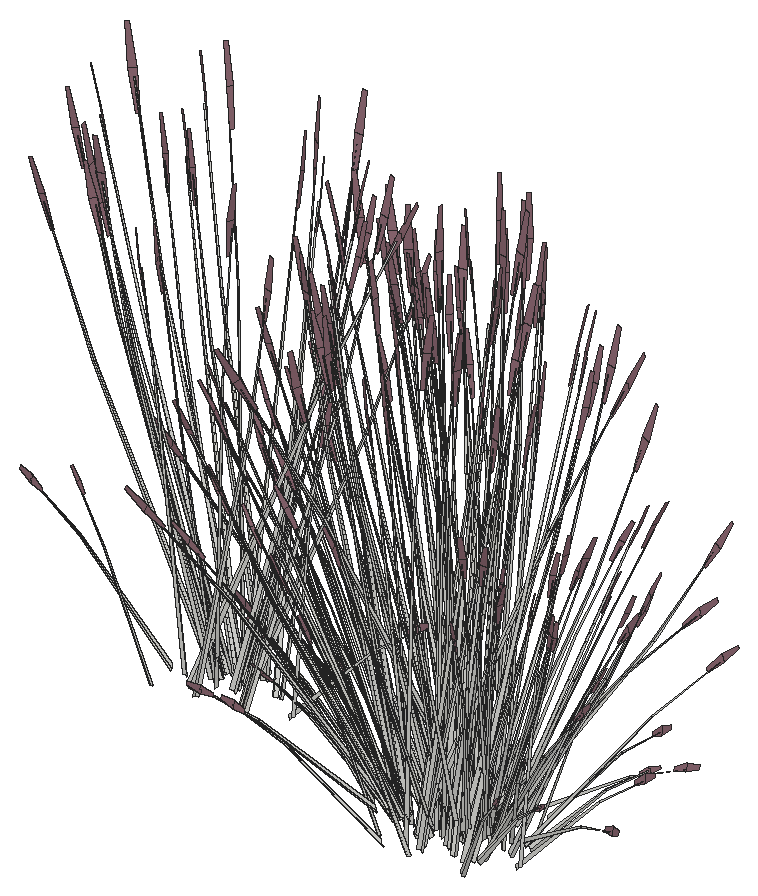
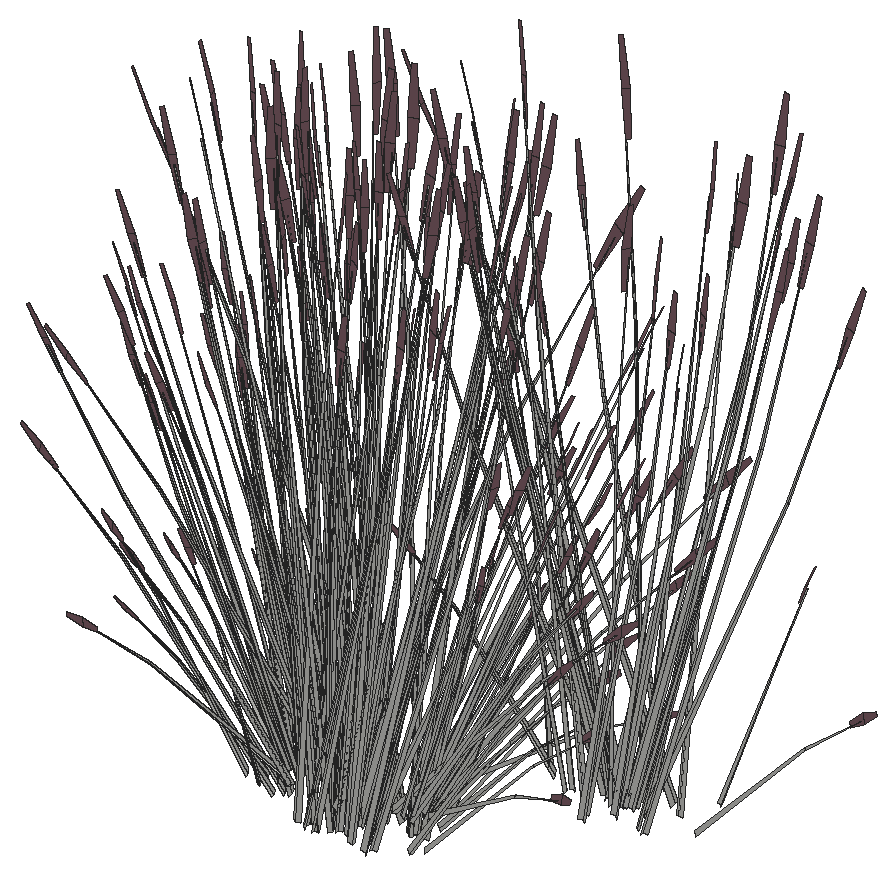
# SketchUp Ruby script. Lengths in inches.
U = 1.inch
M = Sketchup.active_model
def pt(a) = Geom::Point3d.new(a.map { |v| v * U })
def face(e, loops, mat)
  f = e.add_face(loops[0].map { |a| pt(a) })
  loops[1..].each { |l| e.add_face(l.map { |a| pt(a) }).erase! }
  f.material = f.back_material = mat if mat
  f
end
# faces: each face lists its corners as indices into pts; further lists are holes
def faces(e, pts, list, mat = nil) = list.each { |f| face(e, (f[0].is_a?(Array) ? f : [f]).map { |l| l.map { |i| pts[i] } }, mat) }
# xy, xz, yz: faces in a plane at the given z, y or x. An outline is a flat list of corners, or four numbers for a rectangle; further outlines are holes
def ring(l) = l.size == 4 ? [[l[0], l[1]], [l[2], l[1]], [l[2], l[3]], [l[0], l[3]]] : l.each_slice(2).to_a
def flat(e, list, mat, &to3) = list.each { |f| face(e, (f[0].is_a?(Array) ? f : [f]).map { |l| ring(l).map { |u, v| to3.(u, v) } }, mat) }
def xy(e, z, list, mat = nil) = flat(e, list, mat) { |x, y| [x, y, z] }
def xz(e, y, list, mat = nil) = flat(e, list, mat) { |x, z| [x, y, z] }
def yz(e, x, list, mat = nil) = flat(e, list, mat) { |y, z| [x, y, z] }
def lines(e, pts, list) = list.each { |a, b| e.add_line(pt(pts[a]), pt(pts[b])) }
# prism: a flat outline (further loops are holes) pulled along v
def prism(e, loops, v, mat = nil)
  f = face(e, loops, mat); d = Geom::Vector3d.new(v.map { |x| x * U })
  f.pushpull(f.normal.samedirection?(d) ? d.length : -d.length)
end
def box(e, o, s, mat = nil) = prism(e, [[o, [o[0] + s[0], o[1], o[2]], [o[0] + s[0], o[1] + s[1], o[2]], [o[0], o[1] + s[1], o[2]]]], [0, 0, s[2]], mat)
def at(x, y, z, deg = 0) = Geom::Transformation.translation(pt([x, y, z])) * Geom::Transformation.rotation(ORIGIN, Z_AXIS, deg.degrees)
def axes(o, x, y, z) = Geom::Transformation.new([*x, 0, *y, 0, *z, 0, *pt(o).to_a, 1])
def part(name) = M.definitions.add(name)
# library, detail: a bought-in or finely detailed component or shape, given as its bounding box
def library(name, o, s) = part(name).tap { |d| box(d.entities, o, s) }
def detail(e, o, s) = box(e.add_group.entities, o, s)
def put(e, d, t, mat = nil) = e.add_instance(d, t).tap { |i| i.material = mat if mat }
def group(e, t, mat = nil) = e.add_group.tap { |g| g.transformation = t; g.material = mat if mat }.entities
root = M.entities
M.materials.add("LightPink_Translucent").color = [144, 107, 117]
c1 = part("blade")
p = [[2.15,0.21,22],[0,0.17,0],[0.09,0.45,0],[2.18,0.31,22],[2.29,0.31,22],[0.38,0.45,0],
  [2.48,0.24,33],[2.49,0.24,33],[2.48,0.22,33]]
faces(c1.entities,p,[[0,1,2,3],[4,5,2,3],[6,3,4,7],[8,0,3,6]])
c2 = part("seeds")
p = [[0.3,-0.1,1.38],[-0.01,-0.03,1.59],[-0.01,-0.03,0.03],[0.14,-0.07,-0.07],[0.29,-0.03,3],[0.15,0.01,3.11]]
faces(c2.entities,p,[[0,1,2,3],[1,0,4,5]],"LightPink_Translucent")
c3 = part("blade with seeds")
put(c3.entities,c1,at(0,0,0))
put(c3.entities,c2,axes([2.4,0.25,30.99],[1.5799,-0.05474,1.17369],[-0.12525,1.92788,0.29478],[-0.07173,-0.02425,1.56792]))
put(root,c3,axes([73.51,642.17,38.52],[0.55698,-0.6579,0.0643],[0.79316,0.38303,0.50621],[-0.25643,-0.21093,0.77189]))
put(root,c3,axes([71.35,642.08,35.29],[-0.11871,0.13643,1.76342],[-1.19964,0.29415,-0.26939],[-0.2898,-0.26759,0.30037]))
put(root,c3,axes([73.33,645.83,35.89],[-0.50328,-1.06202,-0.69835],[1.44974,-0.38248,-0.18329],[-0.05563,-0.35963,1.54149]))
put(root,c3,axes([70.71,643.46,37.67],[0.45521,0.17844,1.71376],[-0.94204,0.74856,0.13857],[-0.58713,-0.33769,0.73262]))
put(root,c3,axes([80.0625,642.58,35.29],[-0.18342,-0.08159,1.76342],[-0.47115,-0.9115,-0.26939],[0.31784,-0.24736,0.30037]))
put(root,c3,axes([51.08,643.17,44.21],[0.59459,-0.93321,-0.44739],[1.23546,0.44912,0.21531],[0,-0.21512,1.43643]))
put(root,c3,axes([76.27,642.79,38.84],[-0.36946,0.79643,0.35414],[-1.07787,-0.23229,-0.4572],[-0.09883,-0.32066,0.87481]))
put(root,c3,axes([51.625,642.71,44.67],[-0.1428,-1.18174,-0.29095],[1.48733,-0.07145,-0.50002],[0.26191,-0.15741,1.59708]))
put(root,c3,axes([47.9375,642.77,44.03],[0.85545,-0.64616,-0.30978],[0.85545,0.64616,0.30978],[0,-0.20813,1.38974]))
put(root,c3,axes([72.91,642.93,38.47],[-1.20928,0.24619,-0.51099],[-0.21154,-0.93233,-0.3958],[-0.32481,-0.26718,0.97773]))
put(root,c3,axes([79.02,643.125,38.53],[0.87265,0.70663,0.48003],[-0.92674,0.60943,0.3958],[0.16097,-0.33153,0.9933]))
put(root,c3,axes([73.76,642.1,39.22],[-0.81789,0.99285,-0.13619],[-1.18445,-0.572,-0.75594],[-0.41173,-0.28051,1.14864]))
put(root,c3,axes([47.59,639.67,44.13],[-0.35352,0.84566,-0.03893],[-1.08806,-0.26014,-0.17649],[-0.1652,-0.13832,0.58215]))
put(root,c3,axes([79.35,643.19,38.52],[1.00708,0.04826,0.0643],[-0.02761,0.72867,0.50621],[0.10538,-0.27912,0.77189]))
put(root,c3,axes([50.93,643.95,44.67],[-1.38012,-0.49416,-0.29095],[0.66454,-1.04299,-0.50002],[-0.04337,-0.25608,1.59708]))
put(root,c3,axes([78.59,643.6875,38.84],[-0.82919,0.54528,0.35414],[-0.78493,-0.62262,-0.4572],[0.11943,-0.31634,0.87481]))
put(root,c3,axes([80.06,645.16,38.77],[0.64013,-0.81717,-0.71045],[1.12174,0.58074,0.08574],[0.38221,-0.29607,1.00501]))
put(root,c3,axes([51.43,640.09,44.03],[1.14332,0.25625,-0.30978],[-0.28787,0.90242,0.30978],[0.23049,-0.10406,1.38974]))
put(root,c3,axes([73.14,642.78,36.17],[-0.7662,-1.03778,0],[1.28187,-0.57875,-0.51607],[0.29196,-0.13181,1.63711]))
put(root,c3,axes([80.02,644.77,38.47],[-0.31482,-0.94565,-0.51099],[1.19224,-0.16542,-0.3958],[0.34166,-0.254,0.97773]))
put(root,c3,axes([74.82,641.53,35.92],[-0.84686,0.59414,-0.03893],[-0.77596,-0.65071,-0.17649],[-0.05463,-0.18438,0.58215]))
put(root,c3,axes([70.625,641.8125,38.51],[-0.26368,-0.00731,1.74944],[-0.83946,0.73103,-0.27667],[-0.44791,-0.14937,0.14031]))
put(root,c3,axes([80.59,645.45,38.83],[-1.1336,-0.57106,-0.1216],[0.65308,-0.827,-0.67495],[0.32027,-0.28747,1.02557]))
put(root,c3,axes([75.9,648.57,37.12],[1.05902,0.41762,1.51261],[-1.03748,0.89969,0.59816],[-0.46471,-0.53324,1.26806]))
put(root,c3,axes([73.68,642.92,38.84],[0.18927,0.83419,0.35414],[-1.08199,0.22027,-0.4572],[-0.29062,-0.23905,0.87481]))
put(root,c3,axes([70.37,645.68,35.8125],[0,-1.03566,-0.49651],[1.37109,0,0],[0,-0.23588,1.57504]))
put(root,c3,axes([74.18,642.62,35.8125],[1.14694,-0.51783,-0.49651],[0.68554,0.92854,0],[0.26122,-0.11794,1.57504]))
put(root,c3,axes([80.98,644.4,36.38],[-0.4378,-0.03068,1.43002],[-0.44851,-0.8229,-0.30754],[0.53783,-0.23279,0.61141]))
put(root,c3,axes([70.43,643.47,38.89],[1.01205,-0.7643,0.53763],[0.87284,0.81167,0.4433],[-0.47482,-0.14098,1.11249]))
put(root,c3,axes([83.38,645.2,38.5],[-0.16006,-0.00787,1.77383],[-0.66468,-0.8428,-0.16761],[0.26693,-0.27711,0.31391]))
put(root,c3,axes([75.54,644.74,35.85],[0.82544,-0.77843,-0.62353],[1.0254,0.70586,-0.16365],[0.33076,-0.19418,1.37633]))
put(root,c3,axes([51.28,645.04,44.4375],[0.32481,-1.2272,-0.23429],[1.54007,0.21392,0.51271],[-0.26911,-0.16947,1.5644]))
put(root,c3,axes([81.49,642.89,36.56],[-0.40819,0.5272,1.1486],[-0.35086,-0.70831,0.84392],[0.33713,-0.17749,0.25299]))
put(root,c3,axes([80.9,644.87,38.32],[1.06674,-0.14801,-0.35414],[0.28168,0.84611,0.4572],[0.30569,-0.22726,0.87481]))
put(root,c3,axes([70.89,643.46,38.52],[0.06171,-0.78753,0.0643],[0.9318,0.02159,0.50621],[-0.35694,-0.08241,0.77189]))
put(root,c3,axes([74.1,646.1,36],[0.59459,-0.93321,-0.44739],[1.23546,0.44912,0.21531],[0,-0.21512,1.43643]))
put(root,c3,axes([70.54,643.71,38.32],[-0.69728,-0.64842,-0.35414],[0.79619,-0.61382,0.4572],[-0.40453,-0.09339,0.87481]))
put(root,c3,axes([74.64,645.64,36.46],[-0.1428,-1.18174,-0.29095],[1.48733,-0.07145,-0.50002],[0.26191,-0.15741,1.59708]))
put(root,c3,axes([70.95,645.7,35.82],[0.85545,-0.64616,-0.30978],[0.85545,0.64616,0.30978],[0,-0.20813,1.38974]))
put(root,c3,axes([51.17,644.55,44.21],[-0.73619,-0.86927,-0.44739],[1.11511,-0.61213,0.21531],[-0.23824,-0.10756,1.43643]))
put(root,c3,axes([70.61,642.61,35.92],[-0.35352,0.84566,-0.03893],[-1.08806,-0.26014,-0.17649],[-0.1652,-0.13832,0.58215]))
put(root,c3,axes([80.03,645.37,38.84],[-1.06674,0.14801,0.35414],[-0.28168,-0.84611,-0.4572],[0.30569,-0.22726,0.87481]))
put(root,c3,axes([73.95,646.88,36.46],[-1.38012,-0.49416,-0.29095],[0.66454,-1.04299,-0.50002],[-0.04337,-0.25608,1.59708]))
put(root,c3,axes([70.02,646.47,36.17],[-1.53239,0,0],[0,-1.1575,-0.51607],[0,-0.26363,1.63711]))
put(root,c3,axes([60.21,643.33,44.26],[-0.75977,-0.66224,-0.06488],[0.83212,-0.6068,-0.29416],[0.23578,-0.04272,0.97024]))
put(root,c3,axes([70.29,644.4,36.38],[0.23927,0.28834,1.43002],[-0.55135,0.78376,-0.30754],[-0.56612,-0.18733,0.61141]))
put(root,c3,axes([74.45,643.02,35.82],[1.14332,0.25625,-0.30978],[-0.28787,0.90242,0.30978],[0.23049,-0.10406,1.38974]))
put(root,c3,axes([71.27,644.14,38.77],[-1.22504,-0.02494,-0.71045],[0.08228,-1.05005,0.08574],[-0.51899,-0.11081,1.00501]))
put(root,c3,axes([50.51,644.88,44.06],[-1.27479,-0.1698,-0.62353],[0.26901,-1.04736,-0.16365],[-0.38043,-0.12691,1.37633]))
put(root,c3,axes([81,645.24,38.52],[0.8413,0.43556,0.0643],[-0.48981,0.62025,0.50621],[0.26973,-0.20053,0.77189]))
put(root,c3,axes([80.77,645.06,38.53],[0.30393,0.95317,0.48003],[-1.19224,0.16542,0.3958],[0.35138,-0.22417,0.9933]))
put(root,c3,axes([83.98,646.21,38.51],[0.17006,-0.15775,1.74944],[-0.21766,-0.96766,-0.27667],[0.42669,-0.18347,0.14031]))
put(root,c3,axes([50.22,641.94,43.59],[-1.20625,0.41464,1.28929],[-0.38394,-1.1897,0.50096],[0.74071,0.01979,1.46642]))
put(root,c3,axes([71.21,646.16,36.125],[-1.1399,0.87071,0.30756],[-1.1406,-0.86155,-0.36492],[-0.03981,-0.24727,1.64885]))
put(root,c3,axes([69.61,642.43,38.5],[0.09085,0.10335,1.77383],[-0.43798,0.92907,-0.16761],[-0.44357,0.00672,0.31391]))
put(root,c3,axes([59.64,643.56,43.49],[-0.06405,-0.15723,1.76342],[0.44421,-0.91974,-0.26939],[0.4481,-0.01323,0.30037]))
put(root,c3,axes([46.41,643.4,43.49],[0.03108,0.16322,1.76342],[-0.62654,0.85237,-0.26939],[-0.44504,-0.04296,0.30037]))
put(root,c3,axes([74.84,646.57,36.23],[1.3808,0.50196,0.24065],[-0.66454,1.04299,0.50002],[0,-0.24043,1.60543]))
put(root,c3,axes([74.3,647.98,36.23],[0.32481,-1.2272,-0.23429],[1.54007,0.21392,0.51271],[-0.26911,-0.16947,1.5644]))
put(root,c3,axes([49.16,646.47,44.03],[-0.28787,-0.90242,-0.30978],[1.14332,-0.25625,0.30978],[-0.23049,-0.10406,1.38974]))
put(root,c3,axes([70.87,644.36,38.47],[-0.88986,0.68603,-0.51099],[-0.77932,-0.72471,-0.3958],[-0.45212,-0.10438,0.97773]))
put(root,c3,axes([71.53,644.05,38.84],[0.69728,0.64842,0.35414],[-0.79619,0.61382,-0.4572],[-0.40453,-0.09339,0.87481]))
put(root,c3,axes([68.86,645.26,36.56],[0.78239,-0.07411,1.1486],[-0.49629,0.65296,0.84392],[-0.38663,-0.09795,0.25299]))
put(root,c3,axes([53.34,642.56,44.67],[1.23732,-0.68758,-0.29095],[0.8228,0.97154,-0.50002],[0.30528,0.09867,1.59708]))
put(root,c3,axes([48.84,646.86,44.02],[-1.14694,-0.51783,-0.49651],[0.68554,-0.92854,0],[-0.26122,-0.11794,1.57504]))
put(root,c3,axes([74.39,645.87,36.51],[-1.33077,0.06393,0.44739],[-0.12035,-1.06125,-0.21531],[0.23824,-0.10756,1.43643]))
put(root,c3,axes([56.46,640.73,44.02],[1.14694,0.51783,-0.49651],[-0.68554,0.92854,0],[0.26122,0.11794,1.57504]))
put(root,c3,axes([71.33,643.64,38.83],[-0.06562,1.05324,-0.1216],[-1.2424,-0.02879,-0.67495],[-0.4785,-0.07316,1.02557]))
put(root,c3,axes([70.95,646.64,36.27],[0,1.03566,0.49651],[-1.37109,0,0],[0,-0.23588,1.57504]))
put(root,c3,axes([80.63,647.68,38.83],[-0.6166,-0.93779,-0.1216],[1.09436,-0.46085,-0.67495],[0.46117,-0.12373,1.02557]))
put(root,c3,axes([80.58,646.875,38.47],[0.332,-0.94205,-0.51099],[1.13828,0.3229,-0.3958],[0.45829,-0.08638,0.97773]))
put(root,c3,axes([51.96,645.03,44.67],[-1.23732,0.68758,-0.29095],[-0.8228,-0.97154,-0.50002],[-0.30528,-0.09867,1.59708]))
put(root,c3,axes([78.78,643.04,36.17],[0.7662,-1.03778,0],[1.28187,0.57875,-0.51607],[0.29196,0.13181,1.63711]))
put(root,c3,axes([69.75,645.09,37.67],[0.50831,-0.02346,1.71376],[-0.33721,1.01661,0.13857],[-0.72439,-0.06288,0.73262]))
put(root,c3,axes([74.19,647.48,36],[-0.73619,-0.86927,-0.44739],[1.11511,-0.61213,0.21531],[-0.23824,-0.10756,1.43643]))
put(root,c3,axes([74.34,646.25,36.15],[0.53281,1.15808,0.45755],[-1.52239,0.4027,0.17955],[0.01861,-0.2128,1.58856]))
put(root,c3,axes([56.14,641.12,44.03],[0.28787,0.90242,-0.30978],[-1.14332,0.25625,0.30978],[0.23049,0.10406,1.38974]))
put(root,c3,axes([81.79,647.14,35.78],[-0.7893,0.12429,1.41583],[-0.12563,-0.9893,0.08104],[0.55282,-0.14974,0.80566]))
put(root,c3,axes([83.23,646.26,36.05],[-0.75977,-0.66224,-0.06488],[0.83212,-0.6068,-0.29416],[0.23578,-0.04272,0.97024]))
put(root,c3,axes([74.08,647.16,36.51],[-0.59459,0.93321,0.44739],[-1.23546,-0.44912,-0.21531],[0,-0.21512,1.43643]))
put(root,c3,axes([76.26,646.35,36],[0,-1.19833,0],[1.53239,0,0],[0,0,1.79456]))
put(root,c3,axes([78.12,643.58,36.27],[-1.14694,-0.51783,0.49651],[0.68554,-0.92854,0],[0.26122,0.11794,1.57504]))
put(root,c3,axes([80.36,647.22,38.77],[1.07686,-0.45739,-0.71045],[0.60013,0.94154,0.08574],[0.52031,-0.10696,1.00501]))
put(root,c3,axes([73.53,647.8125,35.85],[-1.27479,-0.1698,-0.62353],[0.26901,-1.04736,-0.16365],[-0.38043,-0.12691,1.37633]))
put(root,c3,axes([54.1,646.05,44.18],[1.2866,-0.3514,-0.19198],[0.45209,1.01223,0.00008],[0.14202,-0.03884,1.73897]))
put(root,c3,axes([75.53,645.59,36.15],[-1.01611,0.93987,0.45755],[-1.20717,-0.82966,0.17955],[0.24496,-0.0938,1.58856]))
put(root,c3,axes([76.64,647.28,36.09],[-1.1399,-0.8914,-0.06131],[1.1406,-0.89194,0],[-0.03981,-0.03113,1.75571]))
put(root,c3,axes([73.77,644.05,36.27],[-0.35402,1.02926,0.17642],[-1.29548,-0.29127,0.35086],[0.22379,-0.00501,1.60407]))
put(root,c3,axes([80.2,647.4,38.84],[-1.01846,-0.28891,0.35414],[0.29705,-0.84289,-0.4572],[0.41005,-0.07729,0.87481]))
put(root,c3,axes([54.79,642.71,44.06],[1.27479,0.1698,-0.62353],[-0.26901,1.04736,-0.16365],[0.38043,0.12691,1.37633]))
put(root,c3,axes([69.54,645.86,38.53],[0.34623,-0.9443,0.48003],[1.13828,0.3229,0.3958],[-0.44763,0.05675,0.9933]))
put(root,c3,axes([73.23,644.88,35.39],[-1.20625,0.41464,1.28929],[-0.38394,-1.1897,0.50096],[0.74071,0.01979,1.46642]))
put(root,c3,axes([76.48,645.19,36.41],[0.23642,-0.92427,0.1448],[1.15506,0.16044,-0.41347],[0.21021,0.09491,1.26744]))
put(root,c3,axes([53.35,645.35,44.46],[-1.19666,-0.83357,-0.25192],[1.00694,-0.93603,0.5513],[-0.32224,0.09751,1.68216]))
put(root,c3,axes([69.46,645.61,38.52],[-0.4501,-0.70615,0.0643],[0.82077,-0.34564,0.50621],[-0.36181,0.0682,0.77189]))
put(root,c3,axes([74.48,647.39,36.15],[1.54892,0.2182,0.45755],[-0.31522,1.23236,0.17955],[-0.22636,-0.119,1.58856]))
put(root,c3,axes([82.66,646.49,35.29],[-0.06405,-0.15723,1.76342],[0.44421,-0.91974,-0.26939],[0.4481,-0.01323,0.30037]))
put(root,c3,axes([69.43,646.33,35.29],[0.03108,0.16322,1.76342],[-0.62654,0.85237,-0.26939],[-0.44504,-0.04296,0.30037]))
put(root,c3,axes([75.98,645.43,36.51],[-0.73619,-0.86927,0.44739],[1.11511,-0.61213,-0.21531],[0.23824,0.10756,1.43643]))
put(root,c3,axes([72.18,649.41,35.82],[-0.28787,-0.90242,-0.30978],[1.14332,-0.25625,0.30978],[-0.23049,-0.10406,1.38974]))
put(root,c3,axes([54.125,643.05,44.21],[0.73619,0.86927,-0.44739],[-1.11511,0.61213,0.21531],[0.23824,0.10756,1.43643]))
put(root,c3,axes([73.65,649.35,36.27],[1.31687,-0.27488,0.17642],[0.32517,1.02297,0.35086],[-0.11745,-0.14905,1.60407]))
put(root,c3,axes([76.36,645.49,36.46],[1.23732,-0.68758,-0.29095],[0.8228,0.97154,-0.50002],[0.30528,0.09867,1.59708]))
put(root,c3,axes([81.28,647.3,38.32],[1.01846,0.28891,-0.35414],[-0.29705,0.84289,0.4572],[0.41005,-0.07729,0.87481]))
put(root,c3,axes([71.86,649.79,35.8125],[-1.14694,-0.51783,-0.49651],[0.68554,-0.92854,0],[-0.26122,-0.11794,1.57504]))
put(root,c3,axes([79.48,643.66,35.8125],[1.14694,0.51783,-0.49651],[-0.68554,0.92854,0],[0.26122,0.11794,1.57504]))
put(root,c3,axes([69.31,645.96,38.32],[-1.01846,-0.28891,-0.35414],[0.29705,-0.84289,0.4572],[-0.41005,0.07729,0.87481]))
put(root,c3,axes([77.3,646.62,36],[1.37109,0,0],[0,1.07219,0],[0,0,1.78407]))
put(root,c3,axes([74.98,647.97,36.46],[-1.23732,0.68758,-0.29095],[-0.8228,-0.97154,-0.50002],[-0.30528,-0.09867,1.59708]))
put(root,c3,axes([77.6875,644.1,36.27],[-1.31687,0.27488,0.17642],[-0.32517,-1.02297,0.35086],[0.11745,0.14905,1.60407]))
put(root,c3,axes([52.74,645.17,44.21],[-1.33077,0.06393,-0.44739],[-0.12035,-1.06125,0.21531],[-0.23824,0.10756,1.43643]))
put(root,c3,axes([78.5,646.26,37.67],[-0.50831,0.02346,1.71376],[0.33721,-1.01661,0.13857],[0.72439,0.06288,0.73262]))
put(root,c3,axes([79.16,644.05,35.82],[0.28787,0.90242,-0.30978],[-1.14332,0.25625,0.30978],[0.23049,0.10406,1.38974]))
put(root,c3,axes([81.125,647.66,38.52],[0.4501,0.70615,0.0643],[-0.82077,0.34564,0.50621],[0.36181,-0.0682,0.77189]))
put(root,c3,axes([76.86,646.07,36.17],[-1.54892,-0.2182,0.49198],[0.31522,-1.23236,0.19306],[0.22636,0.119,1.70813]))
put(root,c3,axes([81.04,647.41,38.53],[-0.34623,0.9443,0.48003],[-1.13828,-0.3229,0.3958],[0.44763,-0.05675,0.9933]))
put(root,c3,axes([75.62,649.11,36],[-0.39985,-0.89288,0],[1.1418,-0.31268,0],[0,0,1.54371]))
put(root,c3,axes([74.86,648.27,36.41],[-0.23642,0.92427,0.1448],[-1.15506,-0.16044,-0.41347],[-0.21021,-0.09491,1.26744]))
put(root,c3,axes([70.38,645.87,38.84],[1.01846,0.28891,0.35414],[-0.29705,0.84289,-0.4572],[-0.41005,0.07729,0.87481]))
put(root,c3,axes([77.12,648.99,35.98],[1.2866,-0.3514,-0.19198],[0.45209,1.01223,0.00008],[0.14202,-0.03884,1.73897]))
put(root,c3,axes([77.5625,649.41,36.27],[0.35402,-1.02926,0.17642],[1.29548,0.29127,0.35086],[-0.22379,0.00501,1.60407]))
put(root,c3,axes([77.27,647.08,36.01],[0.85545,0.66896,0],[-0.85545,0.66896,0],[0,0,1.69266]))
put(root,c3,axes([72.41,645.82,37.14],[0.34834,-0.14982,1.77064],[0.12012,1.04605,0.13857],[-0.75452,0.1388,0.63284]))
put(root,c3,axes([79.59,646.78,36.27],[-0.96285,-0.75439,0.17642],[0.97031,-0.7317,0.35086],[-0.10634,0.15406,1.60407]))
put(root,c3,axes([77.8,645.65,35.85],[1.27479,0.1698,-0.62353],[-0.26901,1.04736,-0.16365],[0.38043,0.12691,1.37633]))
put(root,c3,axes([83.4375,647.47,36.56],[-0.75718,0.17097,1.1486],[0.35641,-0.70661,0.84392],[0.40168,0.04835,0.25299]))
put(root,c3,axes([75.34,649.52,35.99],[-1.23546,-0.46496,0],[0.59459,-0.96613,0],[0,0,1.62707]))
put(root,c3,axes([76.37,648.28,36.26],[-1.19666,-0.83357,-0.25192],[1.00694,-0.93603,0.5513],[-0.32224,0.09751,1.68216]))
put(root,c3,axes([73.22,649.875,36.27],[1.14694,0.51783,0.49651],[-0.68554,0.92854,0],[-0.26122,-0.11794,1.57504]))
put(root,c3,axes([53.87,647.5,44.03],[-1.14332,-0.25625,-0.30978],[0.28787,-0.90242,0.30978],[-0.23049,0.10406,1.38974]))
put(root,c3,axes([77.26,646.29,36.51],[0.59459,-0.93321,0.44739],[1.23546,0.44912,-0.21531],[0,0.21512,1.43643]))
put(root,c3,axes([83.08,650.46,38.5],[-0.11081,-0.09067,1.77383],[0.2424,-0.97188,-0.16761],[0.43649,-0.06209,0.31391]))
put(root,c3,axes([54.37,643.64,44.67],[1.38012,0.49416,-0.29095],[-0.66454,1.04299,-0.50002],[0.04337,0.25608,1.59708]))
put(root,c3,axes([68.66,646.52,38.51],[-0.20012,0.13446,1.74944],[0.01702,0.98243,-0.27667],[-0.45871,0.12776,0.14031]))
put(root,c3,axes([77.03,646.83,36.09],[0,1.19774,-0.05637],[-1.53239,0,0],[0,0.03764,1.79368]))
put(root,c3,axes([70,646.39,38.47],[-0.332,0.94205,-0.51099],[-1.13828,-0.3229,-0.3958],[-0.45829,0.08638,0.97773]))
put(root,c3,axes([69.95,645.58,38.83],[0.6166,0.93779,-0.1216],[-1.09436,0.46085,-0.67495],[-0.46117,0.12373,1.02557]))
put(root,c3,axes([77.14,645.98,36],[0.73619,0.86927,-0.44739],[-1.11511,0.61213,0.21531],[0.23824,0.10756,1.43643]))
put(root,c3,axes([82.12,649.65,37.72],[-0.23455,-0.87059,-0.03492],[1.10861,-0.20015,-0.15832],[0.23151,0.05519,0.52218]))
put(root,c3,axes([57.36,644.82,44.03],[-0.85545,0.64616,-0.30978],[-0.85545,-0.64616,0.30978],[0,0.20813,1.38974]))
put(root,c3,axes([72.56,650.42,36.17],[-0.7662,1.03778,0],[-1.28187,-0.57875,-0.51607],[-0.29196,-0.13181,1.63711]))
put(root,c3,axes([79.25,649.63,38.83],[0.06562,-1.05324,-0.1216],[1.2424,0.02879,-0.67495],[0.4785,0.07316,1.02557]))
put(root,c3,axes([53.68,644.88,44.67],[0.1428,1.18174,-0.29095],[-1.48733,0.07145,-0.50002],[-0.26191,0.15741,1.59708]))
put(root,c3,axes([54.22,644.42,44.21],[-0.59459,0.93321,-0.44739],[-1.23546,-0.44912,0.21531],[0,0.21512,1.43643]))
put(root,c3,axes([80.38,646.8125,36.27],[0,-1.03566,0.49651],[1.37109,0,0],[0,0.23588,1.57504]))
put(root,c3,axes([76.94,647.59,36.51],[1.33077,-0.06393,0.44739],[0.12035,1.06125,-0.21531],[-0.23824,0.10756,1.43643]))
put(root,c3,axes([77.77,646.51,36.41],[1.1418,-0.30203,0.1448],[0.39985,0.86246,-0.41347],[0,0.18981,1.26744]))
put(root,c3,axes([79.06,649.21,38.84],[-0.69728,-0.64842,0.35414],[0.79619,-0.61382,-0.4572],[0.40453,0.09339,0.87481]))
put(root,c3,axes([75.76,648.1,36],[-1.33077,0.06393,-0.44739],[-0.12035,-1.06125,0.21531],[-0.23824,0.10756,1.43643]))
put(root,c3,axes([82.02,648.61,36.38],[-0.29514,-0.25472,1.43002],[0.38401,-0.84262,-0.30754],[0.59714,0.11414,0.61141]))
put(root,c3,axes([52.78,645.78,44.06],[-0.82544,0.77843,-0.62353],[-1.0254,-0.70586,-0.16365],[-0.33076,0.19418,1.37633]))
put(root,c3,axes([76.74,649.53,36],[1.23546,0.46496,0],[-0.59459,0.96613,0],[0,0,1.74954]))
put(root,c3,axes([54.14,647.91,44.02],[-1.14694,0.51783,-0.49651],[-0.68554,-0.92854,0],[-0.26122,0.11794,1.57504]))
put(root,c3,axes([57.95,644.84,44.02],[0,1.03566,-0.49651],[-1.37109,0,0],[0,0.23588,1.57504]))
put(root,c3,axes([80.33,649,38.51],[0.26289,-0.01751,1.74944],[0.72108,-0.8046,-0.27667],[0.46761,0.10621,0.14031]))
put(root,c3,axes([77.23,650.5625,35.99],[-0.75665,-1.04141,-0.05142],[1.28187,-0.57875,0.51607],[-0.31588,0.09915,1.6363]))
put(root,c3,axes([76.97,648.04,36.41],[0.90538,0.62224,0.1448],[-0.75521,0.70202,-0.41347],[-0.21021,0.09491,1.26744]))
put(root,c3,axes([69.82,648.21,38.53],[-0.30393,-0.95317,0.48003],[1.19224,-0.16542,0.3958],[-0.35138,0.22417,0.9933]))
put(root,c3,axes([69.58,648.02,38.52],[-0.8413,-0.43556,0.0643],[0.48981,-0.62025,0.50621],[-0.26973,0.20053,0.77189]))
put(root,c3,axes([69.96,646.875,37.67],[0.42521,-0.21906,1.71376],[0.35798,1.01226,0.13857],[-0.66754,0.22878,0.73262]))
put(root,c3,axes([79.31,649.12,38.77],[1.22504,0.02494,-0.71045],[-0.08228,1.05005,0.08574],[0.51899,0.11081,1.00501]))
put(root,c3,axes([77.93,649.96,36.27],[1.14694,-0.51783,0.49651],[0.68554,0.92854,0],[-0.26122,0.11794,1.57504]))
put(root,c3,axes([76.3,649.14,36.08],[0.53281,1.18979,-0.06012],[-1.52239,0.41691,0],[0.01861,0.04155,1.72173]))
put(root,c3,axes([76.89,650.43,35.82],[-1.14332,-0.25625,-0.30978],[0.28787,-0.90242,0.30978],[-0.23049,0.10406,1.38974]))
put(root,c3,axes([68.64,648.6,36.38],[0.42589,0.08502,1.43002],[0.2745,0.86839,-0.30754],[-0.57851,0.16255,0.61141]))
